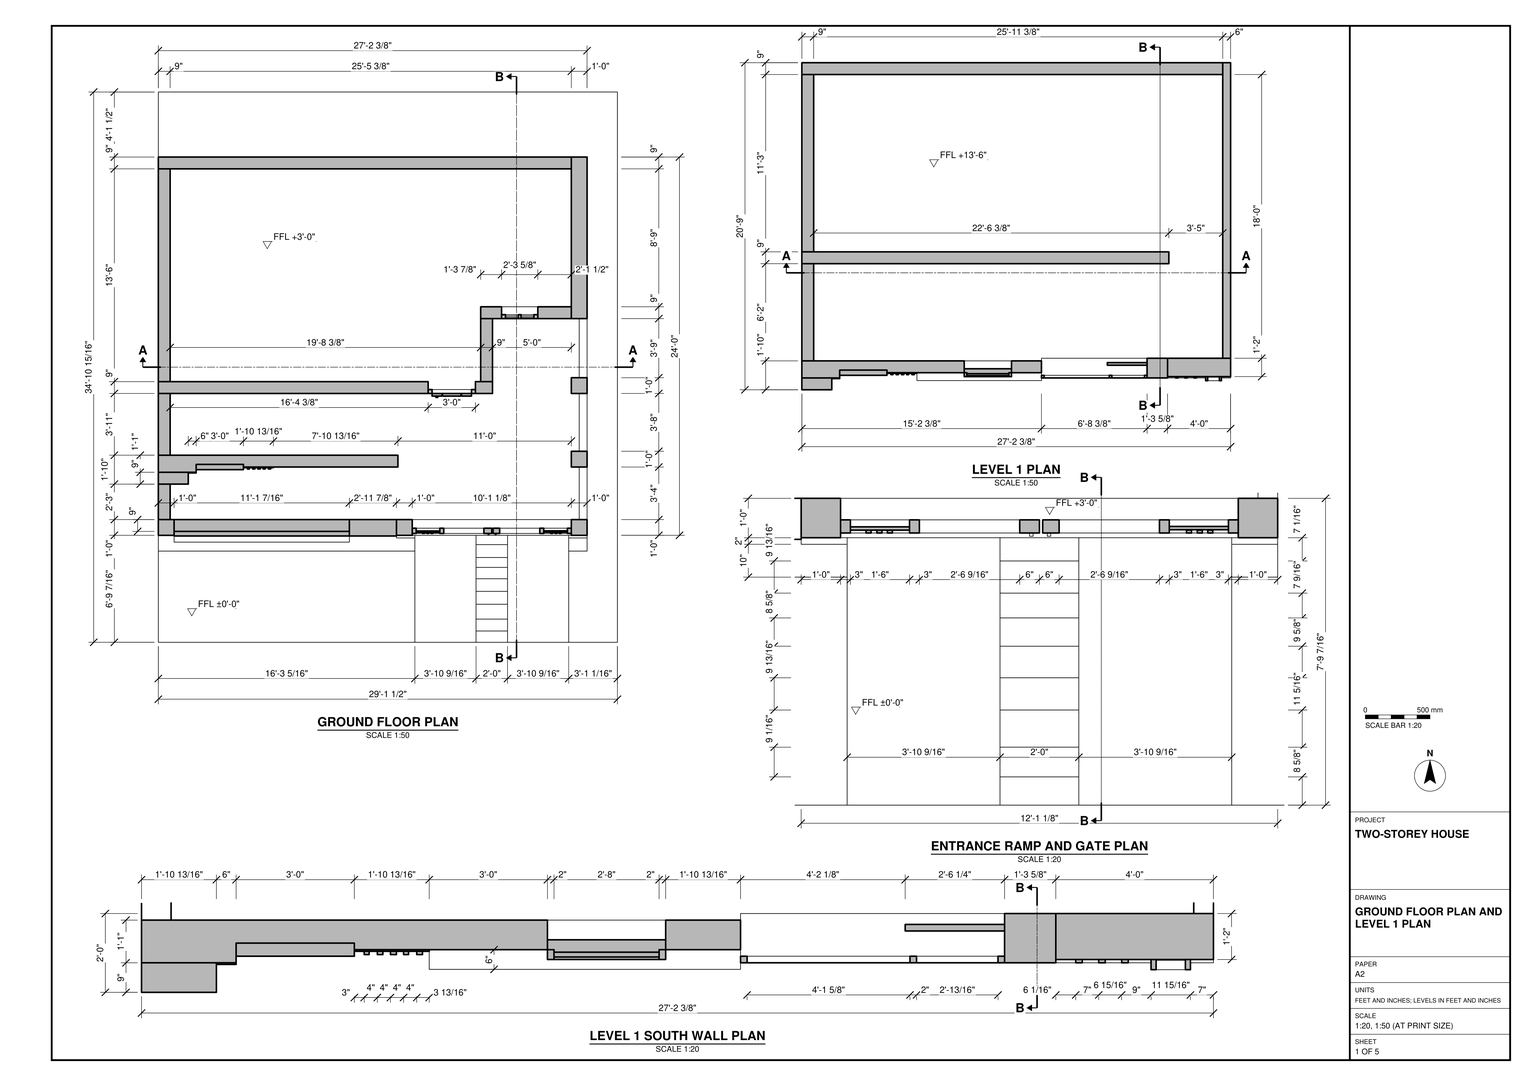
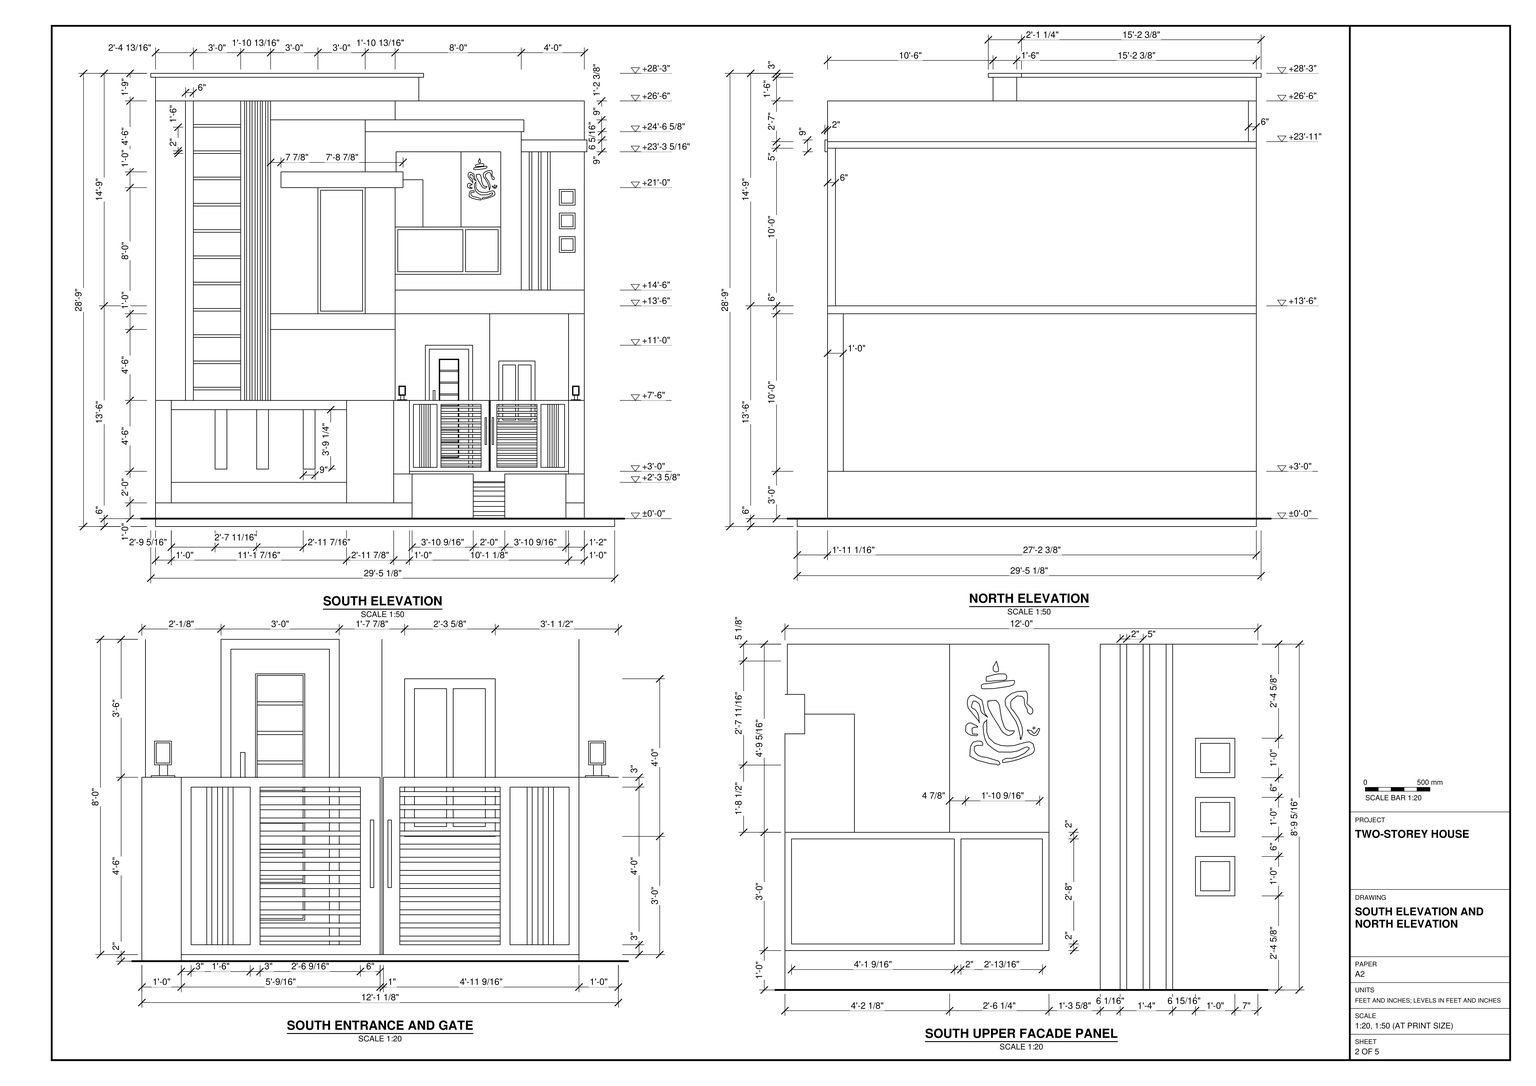
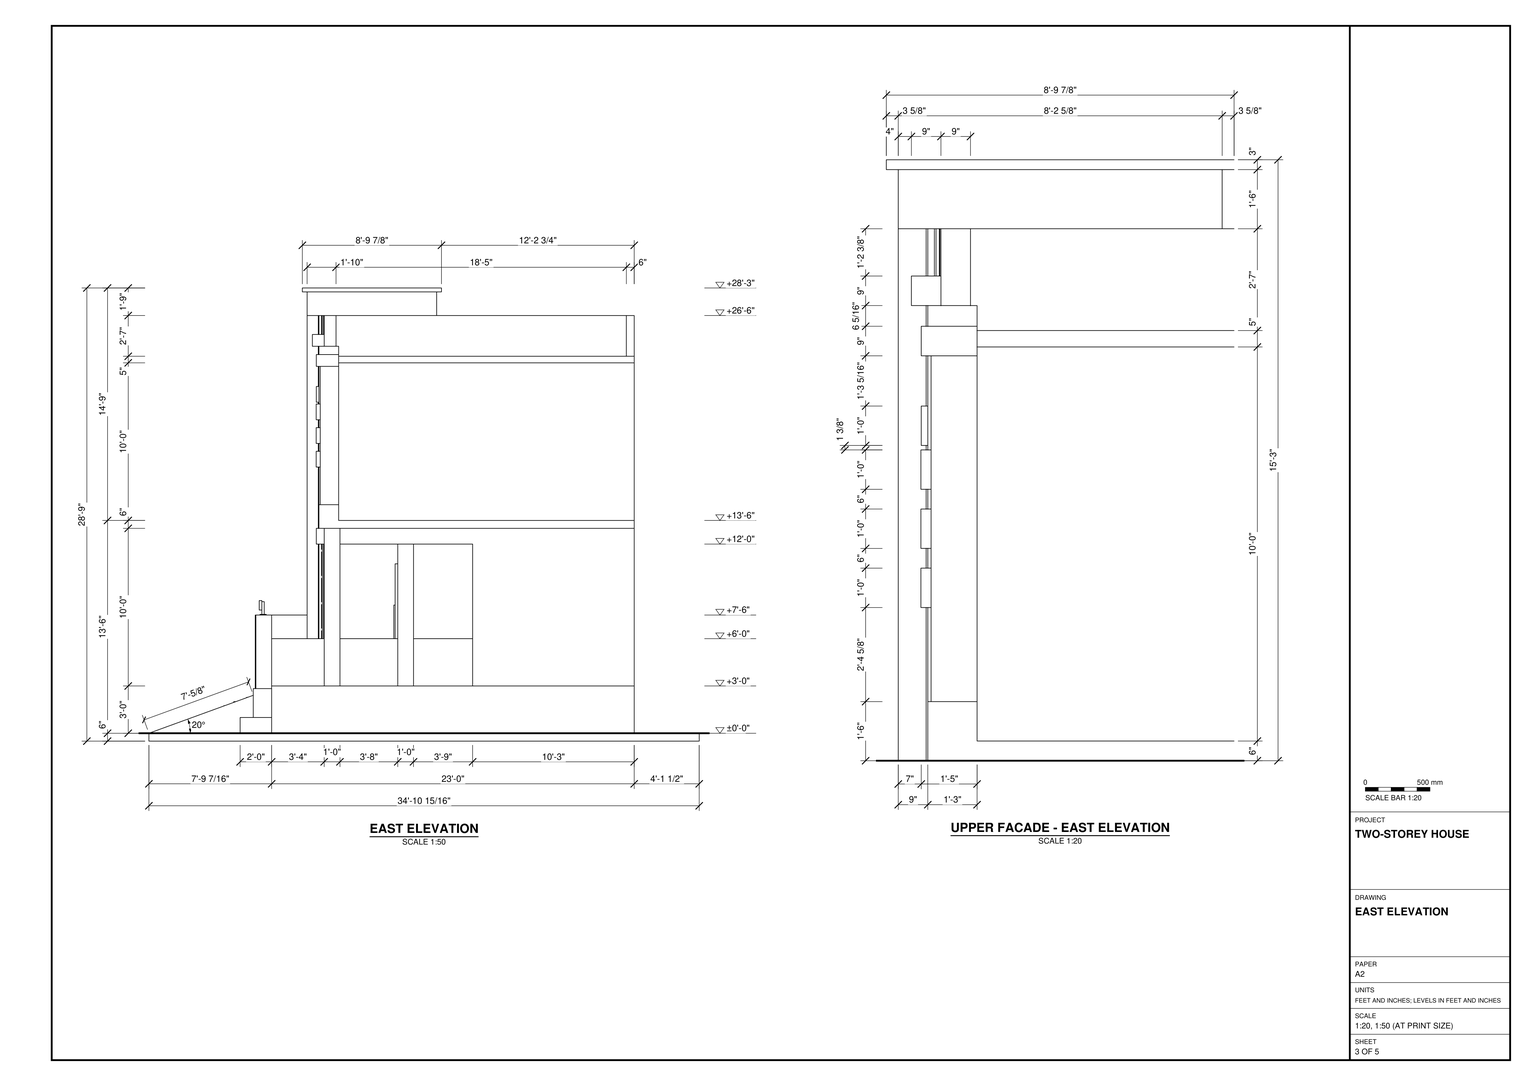
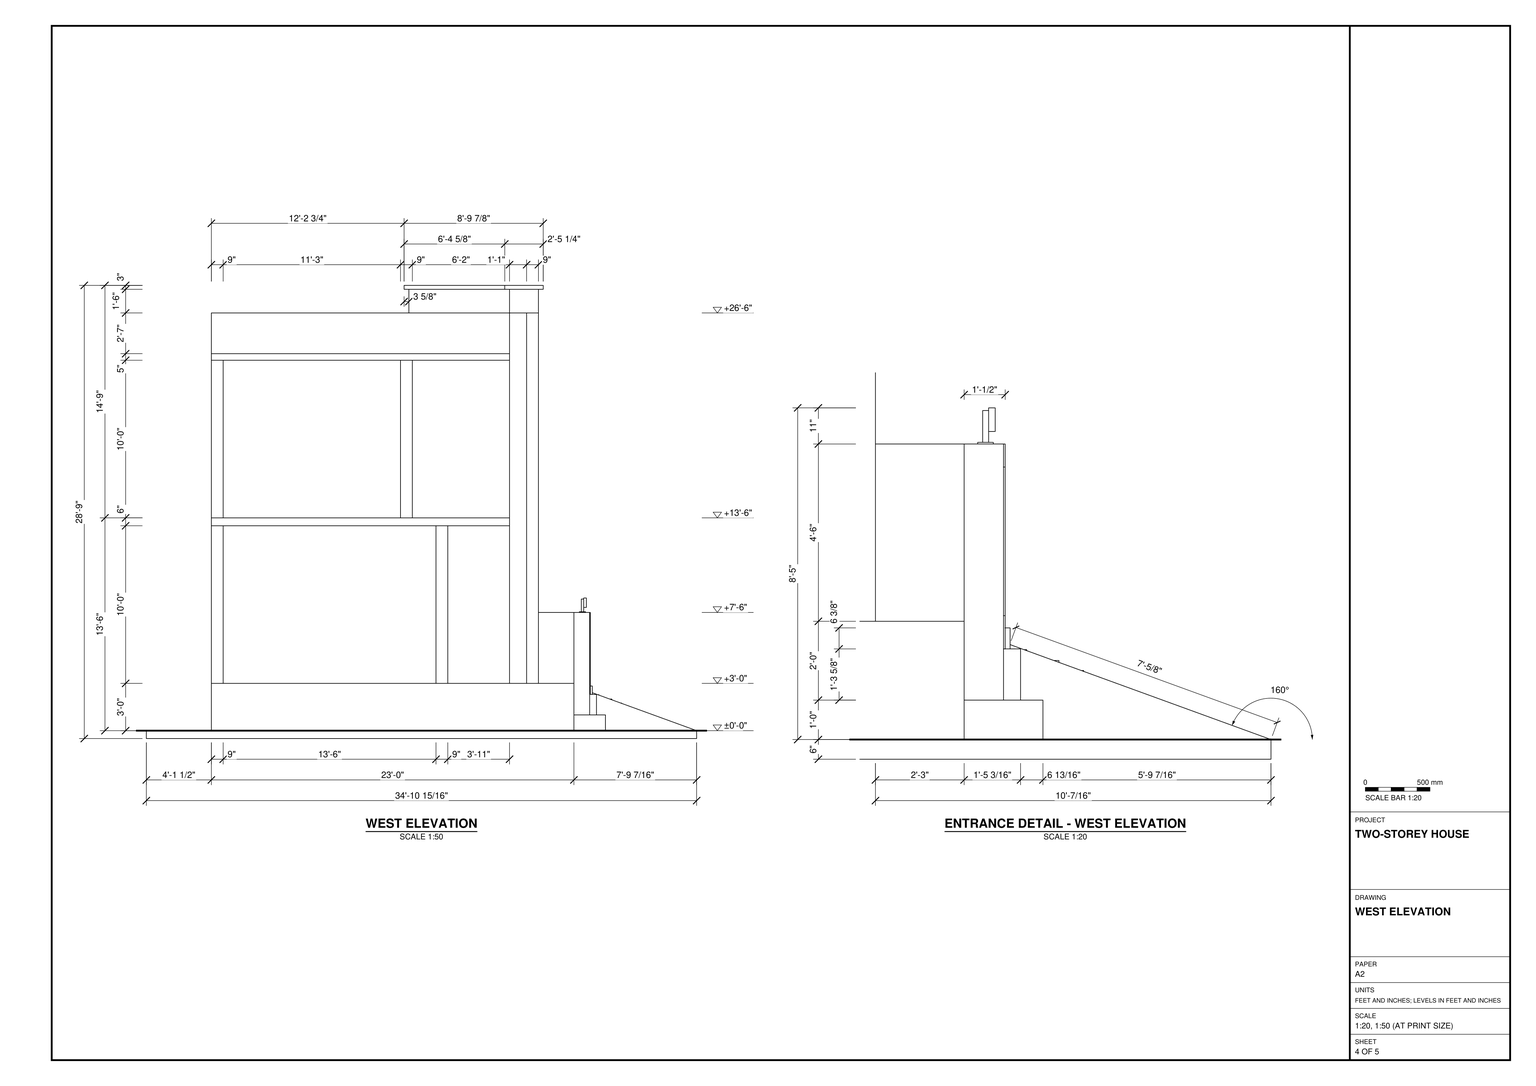
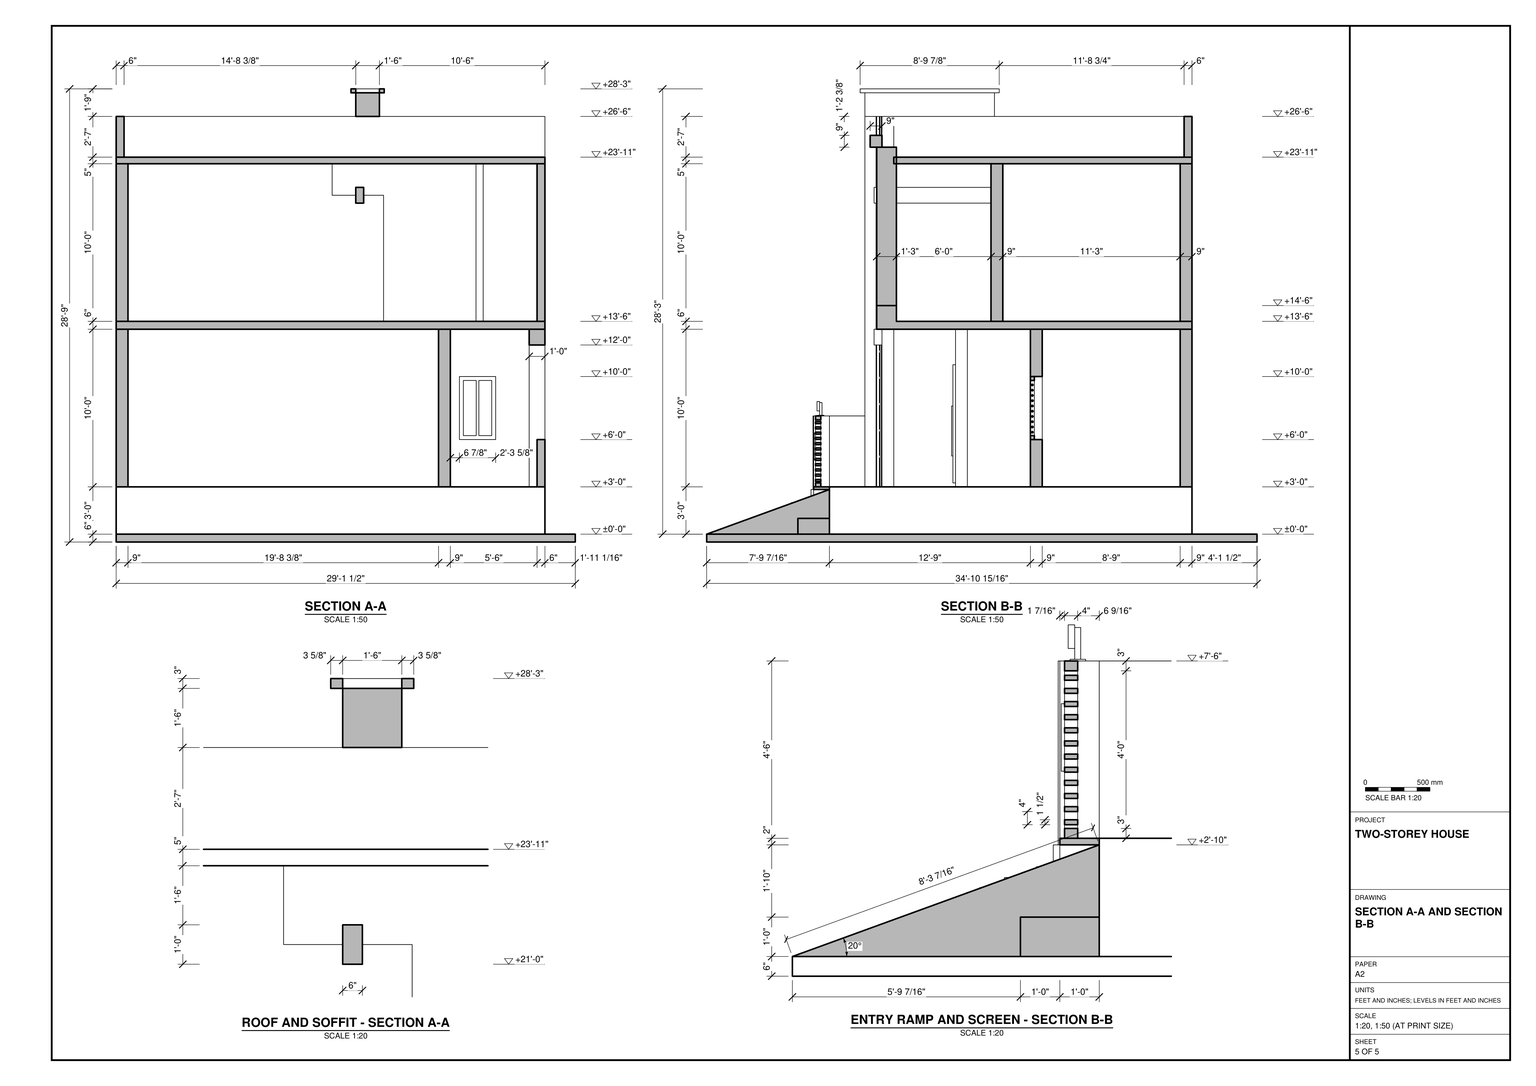
Build the house shown in task_files/diagram_01.pdf in SketchUp. Work in feet and inches, with the south entrance facing the front of the site. Including the base and projecting elements, the overall model must be 29'-5 1/8" wide, 34'-10 15/16" deep and 28'-9" high. Use ±0'-0" as the ground datum and +13'-6" as the upper floor level. The raised lower floor and entrance landing are at +3'-0".

Follow the plans for wall thicknesses, returns, partitions and openings. Model the broad rear room, the recessed entrance area with its posts, and the upper floor with its cross-wall stopping short of the east wall. Include the base, floor slabs, flat roof, parapets and projecting caps. At the south entrance, run the central steps and flanking ramps up to the slatted gate. Set the entrance door and adjacent window back from the gate as drawn.

Use the south elevation for the arrangement of openings, fins and framed panels, and the east elevation for the depths of the projecting bands and hoods. Decor and loose items shown may be represented by any suitable library components. Keep walls, slabs, roof and each furniture or joinery piece shown as separate groups or components, and use components for repeated parts. Save one SketchUp model as output_files/two_storey_house_with_a_gated_entrance.skp.

# SketchUp Ruby script. Lengths in inches.
U = 1.inch
M = Sketchup.active_model
def pt(a) = Geom::Point3d.new(a.map { |v| v * U })
def face(e, loops, mat)
  f = e.add_face(loops[0].map { |a| pt(a) })
  loops[1..].each { |l| e.add_face(l.map { |a| pt(a) }).erase! }
  f.material = f.back_material = mat if mat
  f
end
# faces: each face lists its corners as indices into pts; further lists are holes
def faces(e, pts, list, mat = nil) = list.each { |f| face(e, (f[0].is_a?(Array) ? f : [f]).map { |l| l.map { |i| pts[i] } }, mat) }
# xy, xz, yz: faces in a plane at the given z, y or x. An outline is a flat list of corners, or four numbers for a rectangle; further outlines are holes
def ring(l) = l.size == 4 ? [[l[0], l[1]], [l[2], l[1]], [l[2], l[3]], [l[0], l[3]]] : l.each_slice(2).to_a
def flat(e, list, mat, &to3) = list.each { |f| face(e, (f[0].is_a?(Array) ? f : [f]).map { |l| ring(l).map { |u, v| to3.(u, v) } }, mat) }
def xy(e, z, list, mat = nil) = flat(e, list, mat) { |x, y| [x, y, z] }
def xz(e, y, list, mat = nil) = flat(e, list, mat) { |x, z| [x, y, z] }
def yz(e, x, list, mat = nil) = flat(e, list, mat) { |y, z| [x, y, z] }
def lines(e, pts, list) = list.each { |a, b| e.add_line(pt(pts[a]), pt(pts[b])) }
# prism: a flat outline (further loops are holes) pulled along v
def prism(e, loops, v, mat = nil)
  f = face(e, loops, mat); d = Geom::Vector3d.new(v.map { |x| x * U })
  f.pushpull(f.normal.samedirection?(d) ? d.length : -d.length)
end
def box(e, o, s, mat = nil) = prism(e, [[o, [o[0] + s[0], o[1], o[2]], [o[0] + s[0], o[1] + s[1], o[2]], [o[0], o[1] + s[1], o[2]]]], [0, 0, s[2]], mat)
def at(x, y, z, deg = 0) = Geom::Transformation.translation(pt([x, y, z])) * Geom::Transformation.rotation(ORIGIN, Z_AXIS, deg.degrees)
def axes(o, x, y, z) = Geom::Transformation.new([*x, 0, *y, 0, *z, 0, *pt(o).to_a, 1])
def part(name) = M.definitions.add(name)
# library, detail: a bought-in or finely detailed component or shape, given as its bounding box
def library(name, o, s) = part(name).tap { |d| box(d.entities, o, s) }
def detail(e, o, s) = box(e.add_group.entities, o, s)
def put(e, d, t, mat = nil) = e.add_instance(d, t).tap { |i| i.material = mat if mat }
def group(e, t, mat = nil) = e.add_group.tap { |g| g.transformation = t; g.material = mat if mat }.entities
root = M.entities
M.materials.add("[Blacktop New]").color = [30, 30, 30]
M.materials.add("[Brick Antique 01]2").color = [147, 30, 30]
M.materials.add("[Color A07]").color = [109, 0, 0]
M.materials.add("[Color A07]1").color = [153, 0, 0]
M.materials.add("[Color A08]").color = [102, 0, 0]
M.materials.add("[Color D03]").color = [255, 216, 101]
M.materials.add("[Color E03]").color = [255, 255, 101]
M.materials.add("[Color M00]").color = [255, 255, 255]
M.materials.add("[Color M09]").color = [0, 0, 0]
M.materials.add("[Metal Aluminum Anodized]").color = [202, 209, 219]
M.materials.add("[Polished Concrete New]").color = [200, 200, 203]
M.materials.add("[Translucent Glass Gray]").color = [0, 0, 0]
M.materials["[Translucent Glass Gray]"].alpha = 0.5
c1 = part("Group\#8")
prism(c1.entities,[[[21.6,0.07,0.75],[21.6,0.02,0.63],[21.6,0,0.5],[21.6,0.02,0.37],[21.6,0.07,0.25],[21.6,0.15,0.15],[21.6,0.25,0.07],[21.6,0.37,0.02],[21.6,0.5,0],[21.6,0.63,0.02],[21.6,0.75,0.07],[21.6,0.85,0.15],[21.6,0.93,0.25],[21.6,0.98,0.37],[21.6,1,0.5],[21.6,0.98,0.63],[21.6,0.93,0.75],[21.6,0.85,0.85],[21.6,0.75,0.93],[21.6,0.63,0.98],[21.6,0.5,1],[21.6,0.37,0.98],[21.6,0.25,0.93],[21.6,0.15,0.85]]],[-21.6,0,0])
c2 = part("Group\#17")
prism(c2.entities,[[[32,1.5,0.75],[32,1.47,0.94],[32,1.4,1.125],[32,1.28,1.28],[32,1.125,1.4],[32,0.94,1.47],[32,0.75,1.5],[32,0.56,1.47],[32,0.375,1.4],[32,0.22,1.28],[32,0.1,1.125],[32,0.03,0.94],[32,0,0.75],[32,0.03,0.56],[32,0.1,0.375],[32,0.22,0.22],[32,0.375,0.1],[32,0.56,0.03],[32,0.75,0],[32,0.94,0.03],[32,1.125,0.1],[32,1.28,0.22],[32,1.4,0.375],[32,1.47,0.56]]],[-32,0,0])
c3 = part("Group\#31")
box(c3.entities,[0,0,0],[2,1,105.3])
c4 = part("Group\#67")
box(c4.entities,[0,0,0],[30.55,4,1.5])
c5 = part("Group\#68")
put(c5.entities,c4,at(0,0,44))
put(c5.entities,c4,at(0,0,32))
put(c5.entities,c4,at(0,0,24))
put(c5.entities,c4,at(0,0,12))
put(c5.entities,c4,at(0,0,28))
put(c5.entities,c4,at(0,0,36))
put(c5.entities,c4,at(0,0,16))
put(c5.entities,c4,at(0,0,40))
put(c5.entities,c4,at(0,0,8))
put(c5.entities,c4,at(0,0,20))
put(c5.entities,c4,at(0,0,4))
put(c5.entities,c4,at(0,0,0))
c6 = part("Group\#71")
box(c6.entities,[0,0,0],[1.54,0.875,48])
c7 = part("Group\#72")
put(c7.entities,c6,at(6.49,0,0))
put(c7.entities,c6,at(0,0,0))
put(c7.entities,c6,at(3.3,0,0))
c8 = part("Group\#74")
prism(c8.entities,[[[46.55,93.4375,0],[46.55,93.4375,34],[46.55,0,0],[46.55,69.4375,0]]],[-46.55,0,0])
c9 = part("Group\#84")
box(c9.entities,[0,0,0],[1.0625,1,20.5625])
c10 = library("Group\#47",[0,0,0],[22.59,2.125,31.69])
c11 = part("Group\#91")
xy(c11.entities,0,[[0,0,7.1875,4.75]])
xy(c11.entities,0.5,[[[0,0,7.1875,4.75],[2.48,1.42,4.98,3.23]]])
xy(c11.entities,10.1875,[[2.48,1.42,4.98,3.23]])
xz(c11.entities,0,[[0,0,7.1875,0.5]])
xz(c11.entities,1.42,[[2.48,0.5,4.98,3.8],[2.48,3.8,4.98,10.1875]])
xz(c11.entities,3.23,[[2.48,0.5,4.98,10.1875]])
xz(c11.entities,4.75,[[0,0,7.1875,0.5]])
yz(c11.entities,0,[[0,0,4.75,0.5]])
yz(c11.entities,2.48,[[1.42,0.5,3.23,10.1875]])
yz(c11.entities,4.98,[[1.42,0.5,3.23,10.1875]])
yz(c11.entities,7.1875,[[0,0,4.75,0.5]])
prism(root,[[[99.13,133.4375,258],[186.04,133.4375,258],[186.04,216.4375,258],[192.04,216.4375,258],[192.04,127.4375,258],[99.13,127.4375,258]]],[0,0,12])
xy(root,42,[[3.64,142.4375,12.64,189.4375]])
xy(root,162,[[3.64,142.4375,12.64,189.4375]])
xz(root,142.4375,[[3.64,42,12.64,162]])
xz(root,189.4375,[[3.64,42,12.64,162]])
yz(root,12.64,[[142.4375,42,189.4375,162]])
p = [[186.04,133.4375,258],[186.04,133.4375,257.875],[198.93,69.4375,6],[198.93,69.4375,18],[198.93,79.4375,18],[316.04,69.4375,6],
  [316.04,69.4375,18],[316.04,79.4375,18]]
lines(root,p,[[0,1],[2,3],[3,4],[5,6],[6,7]])
g1 = group(root,at(-29.96,189.4375,42))
prism(g1,[[[288,9,0],[275,9,0],[275,9,96],[239,9,96],[239,9,0],[33.6,9,0],[33.6,9,120],[288,9,120]]],[0,-9,0])
g2 = group(root,at(249.04,198.4375,42))
box(g2,[0,0,0],[9,48,120])
g3 = group(root,at(249.04,246.4375,42))
prism(g3,[[[69,9,0],[0,9,0],[0,9,120],[69,9,120]],[[15.9,9,36],[43.5,9,36],[43.5,9,84],[15.9,9,84]]],[0,-9,0])
g4 = group(root,at(318.04,246.4375,42))
prism(g4,[[[12,0,0],[12,123,0],[12,123,120],[12,-101,120],[12,-101,108],[12,0,108]]],[-12,0,0])
g5 = group(root,at(-29.96,360.4375,42))
box(g5,[33.6,0,0],[314.4,9,120])
g6 = group(root,at(264.9375,246.4375,78),"[Color M09]")
prism(g6,[[[27.6,3,0],[0,3,0],[0,3,48],[27.6,3,48]],[[12.8,3,3],[12.8,3,45],[3,3,45],[3,3,3]],[[24.6,3,45],[14.8,3,45],[14.8,3,3],[24.6,3,3]]],[0,-3,0])
g7 = group(root,at(267.9375,247.4375,83.1))
put(g7,c1,at(0,0,28))
put(g7,c1,at(0,0,36))
put(g7,c1,at(0,0,24))
put(g7,c1,at(0,0,16))
put(g7,c1,at(0,0,12))
put(g7,c1,at(0,0,20))
put(g7,c1,at(0,0,32))
put(g7,c1,at(0,0,0))
put(g7,c1,at(0,0,8))
put(g7,c1,at(0,0,4))
g8 = group(root,at(279.74,246.4375,81),"[Translucent Glass Gray]")
xz(g8,0,[[0,0,9.8,42]])
g9 = group(root,at(267.9375,246.4375,81),"[Translucent Glass Gray]")
xz(g9,0,[[0,0,9.8,42]])
g10 = group(root,at(209.04,189.4375,42),"[Color A07]")
prism(g10,[[[0,0,96],[0,0,0],[36,0,0],[36,0,96]],[[33,0,93],[33,0,3],[3,0,3],[3,0,93]]],[0,3,0])
g11 = group(root,at(212.04,187.4375,45),"[Color A07]")
xy(g11,0,[[0,0,30,2]])
xy(g11,7.5,[[7.5,0,22.5,1]])
xy(g11,8,[[8,0,22,1]])
xy(g11,19,[[8,0,22,0.5]])
xy(g11,20,[[8,0,22,0.5]])
xy(g11,28,[[8,0,22,0.5]])
xy(g11,29,[[8,0,22,0.5]])
xy(g11,37,[[8,0,22,0.5]])
xy(g11,38,[[8,0,22,0.5]])
xy(g11,46,[[8,0,22,0.5]])
xy(g11,47,[[8,0,22,0.5]])
xy(g11,55,[[8,0,22,0.5]])
xy(g11,56,[[8,0,22,0.5]])
xy(g11,64,[[8,0,22,0.5]])
xy(g11,65,[[8,0,22,0.5]])
xy(g11,73,[[8,0,22,0.5]])
xy(g11,74,[[8,0,22,0.5]])
xy(g11,82,[[8,0,22,1]])
xy(g11,82.5,[[7.5,0,22.5,1]])
xy(g11,90,[[0,0,30,2]])
xz(g11,0,[[[0,0,30,90],[7.5,7.5,22.5,82.5]],[8,8,22,19],[8,20,22,28],[8,29,22,37],[8,38,22,46],
  [8,47,22,55],[8,56,22,64],[8,65,22,73],[8,74,22,82]])
xz(g11,0.5,[[8,19,22,20],[8,28,22,29],[8,37,22,38],[8,46,22,47],[8,55,22,56],
  [8,64,22,65],[8,73,22,74]])
xz(g11,1,[[[7.5,7.5,22.5,82.5],[8,8,22,82]]])
xz(g11,2,[[0,0,30,90]])
yz(g11,0,[[0,0,2,90]])
yz(g11,7.5,[[0,7.5,1,82.5]])
yz(g11,8,[[0,8,0,19,0.5,19,0.5,20,0,20,0,28,0.5,28,0.5,29,0,29,0,37,0.5,37,0.5,38,0,38,0,46,0.5,46,0.5,47,0,47,0,55,0.5,55,0.5,56,0,56,0,64,0.5,64,0.5,65,0,65,0,73,0.5,73,0.5,74,0,74,0,82,1,82,1,8]])
yz(g11,22,[[0,8,1,8,1,82,0,82,0,74,0.5,74,0.5,73,0,73,0,65,0.5,65,0.5,64,0,64,0,56,0.5,56,0.5,55,0,55,0,47,0.5,47,0.5,46,0,46,0,38,0.5,38,0.5,37,0,37,0,29,0.5,29,0.5,28,0,28,0,20,0.5,20,0.5,19,0,19]])
yz(g11,22.5,[[0,7.5,1,82.5]])
yz(g11,30,[[0,0,2,90]])
g12 = group(root,at(-29.96,189.4375,162))
xy(g12,0,[[216,-60,216,-47,33.6,-47,33.6,180,360,180,360,-60]])
xy(g12,6,[[33.6,-47,216,-47,216,-45,360,-45,360,180,33.6,180]])
xy(g12,18,[[216,-60,360,-45]])
xz(g12,-60,[[216,0,360,18]])
xz(g12,-47,[[33.6,0,216,6]])
xz(g12,-45,[[216,6,360,18]])
xz(g12,180,[[33.6,0,360,6]])
yz(g12,33.6,[[-47,0,180,6]])
yz(g12,216,[[-60,0,-60,18,-51,18,-51,6,-47,6,-47,0],[-51,6,-45,18]])
yz(g12,360,[[-60,0,180,0,180,6,-45,6,-45,18,-60,18]])
g13 = group(root,at(-29.96,129.4375,42))
xy(g13,0,[[33.6,0,33.6,13,216,13,216,4,98.4,4,98.4,6,62.4,6,62.4,0]])
xy(g13,120,[[157.2,4,193.2,7],[157.2,7,193.2,13]])
xy(g13,216,[[157.2,4,193.2,7],[157.2,7,193.2,13]])
xy(g13,282,[[33.6,0,62.4,0,62.4,6,98.4,6,98.4,4,216,4,216,13,33.6,13]])
xz(g13,0,[[33.6,0,62.4,282]])
xz(g13,4,[[[98.4,0,216,282],[157.2,120,193.2,216]]])
xz(g13,6,[[62.4,0,98.4,282]])
xz(g13,7,[[157.2,120,193.2,216]],"[Color M00]")
xz(g13,13,[[[33.6,0,216,282],[157.2,120,193.2,216]]])
yz(g13,33.6,[[0,0,13,282]])
yz(g13,62.4,[[0,0,6,282]])
yz(g13,98.4,[[4,0,6,282]])
yz(g13,157.2,[[4,120,7,216],[7,120,13,216]])
yz(g13,193.2,[[4,120,7,216],[7,120,13,216]])
yz(g13,216,[[4,0,13,282]])
g14 = group(root,at(127.24,130.4375,162),"[Color M09]")
g15 = group(g14,at(2,0.75,4.64),"[Metal Aluminum Anodized]")
put(g15,c2,at(0,0,54))
put(g15,c2,at(0,0,12))
put(g15,c2,at(0,0,0))
put(g15,c2,at(0,0,42))
put(g15,c2,at(0,0,48))
put(g15,c2,at(0,0,6))
put(g15,c2,at(0,0,30))
put(g15,c2,at(0,0,18))
put(g15,c2,at(0,0,24))
put(g15,c2,at(0,0,36))
put(g15,c2,at(0,0,84))
put(g15,c2,at(0,0,60))
put(g15,c2,at(0,0,78))
put(g15,c2,at(0,0,72))
put(g15,c2,at(0,0,66))
g16 = group(g14,at(0,0,0))
prism(g16,[[[36,0,0],[36,0,96],[0,0,96],[0,0,0]],[[2,0,94],[34,0,94],[34,0,2],[2,0,2]]],[0,3,0])
g17 = group(root,at(129.24,130.4375,164),"[Translucent Glass Gray]")
xz(g17,0,[[0,0,32,92]],"[Translucent Glass Gray]")
g18 = group(root,at(32.4375,132.4375,42),"[Polished Concrete New]")
prism(g18,[[[36,3,0],[36,3,282],[36,-1,282],[36,-1,264],[36,-0.5,264],[36,-0.5,262],[36,-1,262],[36,-1,244],[36,-0.5,244],[36,-0.5,242],[36,-1,242],[36,-1,224],[36,-0.5,224],[36,-0.5,222],[36,-1,222],[36,-1,204],[36,-0.5,204],[36,-0.5,202],[36,-1,202],[36,-1,184],[36,-0.5,184],[36,-0.5,182],[36,-1,182],[36,-1,164],[36,-0.5,164],[36,-0.5,162],[36,-1,162],[36,-1,144],[36,-0.5,144],[36,-0.5,142],[36,-1,142],[36,-1,124],[36,-0.5,124],[36,-0.5,122],[36,-1,122],[36,-1,104],[36,-0.5,104],[36,-0.5,102],[36,-1,102],[36,-1,84],[36,-0.5,84],[36,-0.5,82],[36,-1,82],[36,-1,64],[36,-0.5,64],[36,-0.5,62],[36,-1,62],[36,-1,44],[36,-0.5,44],[36,-0.5,42],[36,-1,42],[36,-1,24],[36,-0.5,24],[36,-0.5,22],[36,-1,22],[36,-1,0]]],[-36,0,0])
g19 = group(root,at(-29.96,129.4375,30))
box(g19,[33.6,-36,-24],[326.4,276,36])
g20 = group(root,at(26.4375,128.9375,42),"[Color A07]")
box(g20,[0,0,0],[6,0.5,282])
g21 = group(root,at(68.4375,132.9375,42))
box(g21,[0,0,0],[22.8,0.5,282],"[Color A07]")
g22 = group(root,at(71.4375,131.9375,42))
box(g22,[0,0,0],[1.5,1,282])
g23 = group(root,at(75.4375,131.9375,42))
box(g23,[0,0,0],[1.6875,1,282])
g24 = group(root,at(79.4375,131.9375,42))
box(g24,[0,0,0],[1.8125,1,282])
g25 = group(root,at(83.4375,131.9375,42))
box(g25,[0,0,0],[1.5,1,282])
g26 = group(root,at(87.4375,131.9375,42))
box(g26,[0,0,0],[1.75,1,282])
g27 = group(root,at(91.24,127.4375,150))
box(g27,[0,0,0],[94.8,6,12])
g28 = group(root,at(163.24,128.4375,270),"[Color A07]")
prism(g28,[[[0,16,30.6],[118.8,16,30.6],[118.8,16,-90],[22.8,16,-90],[22.8,16,-78],[103.2,16,-78],[103.2,16,15.3],[23.53,16,15.3],[23.53,16,0],[0,16,0]]],[0,-15,0])
g29 = group(root,at(282.04,130.4375,180))
box(g29,[0,0,0],[48,14,105.3],"[Color A07]")
g30 = group(root,at(163.24,124.4375,300.6))
box(g30,[0,0,0],[120.8,9,9])
g31 = group(root,at(282.04,127.4375,285.3))
box(g31,[0,0,0],[50,17,9])
put(root,c3,at(288.1,129.4375,180))
put(root,c3,at(295.1,129.4375,180))
put(root,c3,at(302.1,129.4375,180))
g32 = group(root,at(311.04,127.34,226.65))
xy(g32,0,[[0,0,12,3.1]])
xy(g32,1.55,[[1.55,0,10.45,3]])
xy(g32,10.45,[[1.55,0,10.45,3]])
xy(g32,12,[[0,0,12,3.1]])
xz(g32,0,[[[0,0,12,12],[1.55,1.55,10.45,10.45]]])
xz(g32,3,[[1.55,1.55,10.45,10.45]],"[Color D03]")
xz(g32,3.1,[[[0,0,12,12],[1.55,1.55,10.45,10.45]]])
yz(g32,0,[[0,0,3.1,12]])
yz(g32,1.55,[[0,1.55,3,10.45]])
yz(g32,10.45,[[0,1.55,3,10.45]])
yz(g32,12,[[0,0,3.1,12]])
p = [[10.45,3.1,10.45],[10.45,3,10.45],[1.55,3.1,1.55],[1.55,3,1.55],[1.55,3.1,10.45],[1.55,3,10.45],
  [10.45,3.1,1.55],[10.45,3,1.55]]
lines(g32,p,[[0,1],[2,3],[4,5],[6,7]])
g33 = group(root,at(311.04,127.34,208.65))
xy(g33,0,[[0,0,12,3.1]],"[Color D03]")
xy(g33,1.55,[[1.55,0,10.45,3]],"[Color D03]")
xy(g33,10.45,[[1.55,0,10.45,3]],"[Color D03]")
xy(g33,12,[[0,0,12,3.1]],"[Color D03]")
xz(g33,0,[[[0,0,12,12],[1.55,1.55,10.45,10.45]]],"[Color D03]")
xz(g33,3,[[1.55,1.55,10.45,10.45]],"[Color D03]")
xz(g33,3.1,[[[0,0,12,12],[1.55,1.55,10.45,10.45]]],"[Color D03]")
yz(g33,0,[[0,0,3.1,12]],"[Color D03]")
yz(g33,1.55,[[0,1.55,3,10.45]],"[Color D03]")
yz(g33,10.45,[[0,1.55,3,10.45]],"[Color D03]")
yz(g33,12,[[0,0,3.1,12]],"[Color D03]")
p = [[10.45,3.1,10.45],[10.45,3,10.45],[1.55,3.1,1.55],[1.55,3,1.55],[1.55,3.1,10.45],[1.55,3,10.45],
  [10.45,3.1,1.55],[10.45,3,1.55]]
lines(g33,p,[[0,1],[2,3],[4,5],[6,7]])
g34 = group(root,at(311.04,127.34,244.65))
xy(g34,0,[[0,0,12,3.1]])
xy(g34,1.55,[[1.55,0,10.45,3]])
xy(g34,10.45,[[1.55,0,10.45,3]])
xy(g34,12,[[0,0,12,3.1]])
xz(g34,0,[[[0,0,12,12],[1.55,1.55,10.45,10.45]]])
xz(g34,3,[[1.55,1.55,10.45,10.45]],"[Color D03]")
xz(g34,3.1,[[[0,0,12,12],[1.55,1.55,10.45,10.45]]])
yz(g34,0,[[0,0,3.1,12]])
yz(g34,1.55,[[0,1.55,3,10.45]])
yz(g34,10.45,[[0,1.55,3,10.45]])
yz(g34,12,[[0,0,3.1,12]])
p = [[10.45,3.1,10.45],[10.45,3,10.45],[1.55,3.1,1.55],[1.55,3,1.55],[1.55,3.1,10.45],[1.55,3,10.45],
  [10.45,3.1,1.55],[10.45,3,1.55]]
lines(g34,p,[[0,1],[2,3],[4,5],[6,7]])
g35 = group(root,at(91.24,133.14,309.6),"[Color A07]")
box(g35,[0,0,0],[94.8,0.3,14.4])
g36 = group(root,at(3.64,120.4375,42))
box(g36,[0,0,0],[22.8,9,282])
g37 = group(root,at(0,116.8,324))
xy(g37,0,[[3.64,3.64,3.64,25.64,186.04,25.64,186.04,102.26,204.04,102.26,204.04,3.64]])
xy(g37,18,[[[0,0,0,29.27,182.4,29.27,182.4,105.9,207.67,105.9,207.67,0],[3.64,3.64,204.04,3.64,204.04,102.26,186.04,102.26,186.04,25.64,3.64,25.64]],[3.64,3.64,204.04,3.64,204.04,102.26,186.04,102.26,186.04,25.64,3.64,25.64]])
xy(g37,21,[[[0,0,207.67,0,207.67,105.9,182.4,105.9,182.4,29.27,0,29.27],[3.64,3.64,3.64,25.64,186.04,25.64,186.04,102.26,204.04,102.26,204.04,3.64]]],"[Color A08]")
xz(g37,0,[[0,18,207.67,21]],"[Color A08]")
xz(g37,3.64,[[3.64,0,204.04,18]])
xz(g37,3.64,[[3.64,18,204.04,21]],"[Color A08]")
xz(g37,25.64,[[3.64,0,186.04,18]])
xz(g37,25.64,[[3.64,18,186.04,21]],"[Color A08]")
xz(g37,29.27,[[0,18,182.4,21]],"[Color A08]")
xz(g37,102.26,[[186.04,0,204.04,18]])
xz(g37,102.26,[[186.04,18,204.04,21]],"[Color A08]")
xz(g37,105.9,[[182.4,18,207.67,21]])
yz(g37,0,[[0,18,29.27,21]],"[Color A08]")
yz(g37,3.64,[[3.64,0,25.64,18],[3.64,18,25.64,21]])
yz(g37,182.4,[[29.27,18,105.9,21]],"[Color A08]")
yz(g37,186.04,[[25.64,0,102.26,18]])
yz(g37,186.04,[[25.64,18,102.26,21]],"[Color A08]")
yz(g37,204.04,[[3.64,0,102.26,18]])
yz(g37,204.04,[[3.64,18,102.26,21]],"[Color A08]")
yz(g37,207.67,[[0,18,105.9,21]],"[Color A08]")
g38 = group(root,at(3.64,216.4375,168))
xy(g38,0,[[0,0,279.39,9]])
xy(g38,120,[[0,0,279.39,9]])
xz(g38,0,[[0,0,203.55,0,203.55,96,164.4,96,164.4,120,0,120],[273.93,0,279.39,120]])
xz(g38,0,[[203.55,0,273.93,0,273.93,120,164.4,120,164.4,96,203.55,96]],"[Brick Antique 01]2")
xz(g38,9,[[0,0,279.39,120]])
yz(g38,0,[[0,0,9,120]])
yz(g38,279.39,[[0,0,9,120]])
g39 = group(root,at(3.64,144.4375,168))
xy(g39,0,[[320.4,0,326.4,225],[0,216,320.4,225]])
xy(g39,120,[[320.4,0,326.4,225],[0,216,320.4,225]])
xz(g39,0,[[320.4,0,326.4,120]])
xz(g39,216,[[0,0,320.4,120]])
xz(g39,225,[[0,0,320.4,120],[320.4,0,326.4,120]])
yz(g39,0,[[216,0,225,120]])
yz(g39,320.4,[[0,0,216,120],[216,0,225,120]])
yz(g39,326.4,[[0,0,225,120]])
g40 = group(root,at(3.64,225.4375,168))
box(g40,[0,0,0],[9,135,120])
g41 = group(root,at(3.64,198.4375,42))
box(g41,[0,0,0],[9,162,120])
g42 = group(root,at(3.64,142.4375,42))
yz(g42,0,[[0,0,47,120]])
g43 = group(root,at(3.64,142.4375,168))
box(g43,[0,0,0],[9,74,120])
g44 = group(root,at(3.64,142.4375,288))
xy(g44,0,[[0,0,326.4,227]],"[Color E03]")
xy(g44,5,[[0,0,326.4,227]])
xz(g44,0,[[0,0,326.4,5]])
xz(g44,227,[[0,0,326.4,5]])
yz(g44,0,[[0,0,227,5]])
yz(g44,326.4,[[0,0,227,5]])
g45 = group(root,at(186.04,129.4375,192),"[Color M09]")
prism(g45,[[[0,2,0],[0,2,36],[80.4,2,36],[80.4,2,0]],[[51.59,2,34],[2,2,34],[2,2,2],[51.59,2,2]],[[53.59,2,34],[53.59,2,2],[78.4,2,2],[78.4,2,34]]],[0,-2,0])
g46 = group(root,at(239.625,129.4375,194),"[Translucent Glass Gray]")
xz(g46,0,[[0,0,24.81,32]])
g47 = group(root,at(188.04,129.4375,194),"[Translucent Glass Gray]")
xz(g47,0,[[0,0,49.59,32]])
g48 = group(root,at(318.04,133.4375,42))
box(g48,[0,0,0],[12,12,120])
g49 = group(root,at(318.04,189.4375,42))
box(g49,[0,0,0],[12,12,108])
g50 = group(root,at(-18.9375,0,0))
box(g50,[22.57,0,0],[349.49,418.9375,6])
g51 = group(root,at(3.64,69.4375,6))
box(g51,[0,0,0],[326.4,24,12])
g52 = group(root,at(3.64,81.4375,18))
box(g52,[0,0,0],[12,12,78])
g53 = group(root,at(15.64,76.25,18))
box(g53,[0,0,0],[133.4375,17.1875,15.6])
g54 = group(root,at(15.64,84.4375,33.6))
box(g54,[0,0,0],[133.4375,9,56.4])
g55 = group(root,at(15.64,80.9375,88.98))
box(g55,[0,0,0],[133.4375,12.5,7.03])
g56 = group(root,at(48.95,80.9375,43.72),"[Color A07]")
box(g56,[0,0,0],[9,3.5,45.25])
g57 = group(root,at(80.64,80.9375,43.72),"[Color A07]")
box(g57,[0,0,0],[9,3.5,45.25])
g58 = group(root,at(116.07,80.9375,43.72),"[Color A07]")
box(g58,[0,0,0],[9,3.5,45.25])
g59 = group(root,at(149.07,80.9375,18),"[Color A07]")
box(g59,[0,0,0],[35.86,12.5,78])
g60 = group(root,at(184.93,79.4375,18))
box(g60,[0,0,0],[14,14,22])
g61 = group(root,at(316.04,79.4375,18))
box(g61,[0,0,0],[14,14,22])
g62 = group(root,at(184.93,81.4375,42))
box(g62,[0,0,-2],[12,12,56])
g63 = group(root,at(318.04,81.4375,42))
box(g63,[0,0,-2],[12,12,56])
g64 = group(root,at(196.93,81.4375,40),"[Color A08]")
prism(g64,[[[0,12,2],[121.1,12,2],[121.1,12,0],[72.55,12,0],[72.55,12,-5.88],[48.55,12,-5.88],[48.55,12,0],[0,12,0]]],[0,-12,0])
g65 = group(root,at(196.93,82.875,42))
put(g65,c5,at(24,0,4.11),"[Color M09]")
g66 = group(g65,at(0,0,0),"[Color M09]")
prism(g66,[[[60.55,0,54],[0,0,54],[0,0,0],[60.55,0,0]],[[24,0,3],[24,0,51],[54.55,0,51],[54.55,0,3]],[[21,0,3],[3,0,3],[3,0,51],[21,0,51]]],[0,4,0])
g67 = group(g65,at(61.55,0,0),"[Color M09]")
prism(g67,[[[59.55,4,0],[0,4,0],[0,4,54],[59.55,4,54]],[[35.55,4,3],[35.55,4,51],[5,4,51],[5,4,3]],[[56.55,4,51],[38.55,4,51],[38.55,4,3],[56.55,4,3]]],[0,-4,0])
g68 = group(g65,at(100.1,1,3))
box(g68,[0,0,0],[18,1,48],"[Color A07]")
g69 = group(g65,at(3,0.875,3))
box(g69,[0,0,0],[18,1,48],"[Color A07]")
put(g65,c7,at(7.76,0,3))
put(g65,c7,at(105.32,0,3))
put(g65,c5,at(66.55,0,4.14),"[Color M09]")
put(root,c8,at(198.93,0,6),"[Color A07]1")
put(root,c8,at(269.48,0,6),"[Color A07]1")
g70 = group(root,at(245.48,0,6),"[Color A08]")
xy(g70,0,[[0,0,24,8.61],[0,8.61,24,17.66],[0,17.66,24,28.97],[0,28.97,24,38.79],[0,38.79,24,48.39],
  [0,48.39,24,61.15],[0,61.15,24,69.4375]])
xy(g70,0.1875,[[0,0,24,8.61]])
xy(g70,2.25,[[0,8.61,24,17.66]])
xy(g70,5.4375,[[0,17.66,24,28.97]])
xy(g70,9.3125,[[0,28.97,24,38.79]])
xy(g70,12,[[0,69.4375,24,79.55],[0,79.55,24,93.4375]])
xy(g70,13.0625,[[0,38.79,24,48.39]])
xy(g70,17.125,[[0,48.39,24,57.02],[0,57.02,24,61.15]])
xy(g70,21,[[0,57.02,24,64.5625],[0,64.5625,24,69.4375]])
xy(g70,24.0625,[[0,64.5625,24,74.36],[0,74.36,24,79.55]])
xy(g70,27.36,[[0,74.36,24,93.4375]])
xz(g70,0,[[0,0,24,0.1875]])
xz(g70,8.61,[[0,0,24,0.1875],[0,0.1875,24,2.25]])
xz(g70,17.66,[[0,0,24,2.25],[0,2.25,24,5.4375]])
xz(g70,28.97,[[0,0,24,5.4375],[0,5.4375,24,9.3125]])
xz(g70,38.79,[[0,0,24,9.3125],[0,9.3125,24,13.0625]])
xz(g70,48.39,[[0,0,24,13.0625],[0,13.0625,24,17.125]])
xz(g70,57.02,[[0,17.125,24,21]])
xz(g70,61.15,[[0,0,24,17.125]])
xz(g70,64.5625,[[0,21,24,24.0625]])
xz(g70,69.4375,[[0,0,24,12],[0,12,24,21]])
xz(g70,74.36,[[0,24.0625,24,27.36]])
xz(g70,79.55,[[0,12,24,24.0625]])
xz(g70,93.4375,[[0,12,24,27.36]])
yz(g70,0,[[0,0,8.61,0.1875],[8.61,0,17.66,2.25],[17.66,0,28.97,5.4375],[28.97,0,38.79,9.3125],[38.79,0,48.39,13.0625],
  [48.39,0,61.15,17.125],[61.15,0,61.15,17.125,57.02,17.125,57.02,21,69.4375,21,69.4375,0],[69.4375,12,69.4375,21,64.5625,21,64.5625,24.0625,79.55,24.0625,79.55,12],[79.55,12,79.55,24.0625,74.36,24.0625,74.36,27.36,93.4375,27.36,93.4375,12]])
yz(g70,24,[[0,0,8.61,0.1875],[8.61,0,17.66,2.25],[17.66,0,28.97,5.4375],[28.97,0,38.79,9.3125],[38.79,0,48.39,13.0625],
  [48.39,0,61.15,17.125],[61.15,0,69.4375,0,69.4375,21,57.02,21,57.02,17.125,61.15,17.125],[69.4375,12,79.55,12,79.55,24.0625,64.5625,24.0625,64.5625,21,69.4375,21],[79.55,12,93.4375,12,93.4375,27.36,74.36,27.36,74.36,24.0625,79.55,24.0625]])
g71 = group(root,at(214.97,186.4375,65.55))
box(g71,[0,0,0],[1.375,1,38])
g72 = group(root,at(3.64,93.4375,42))
box(g72,[0,0,0],[9,27,54])
put(root,c9,at(259.87,81.875,62.42))
put(root,c9,at(254.49,81.875,62.42))
g73 = group(root,at(324.04,93.4375,42))
box(g73,[0,0,0],[6,40,36])
g74 = group(root,at(324.04,145.4375,42))
box(g74,[0,0,0],[6,44,36])
g75 = group(root,at(324.04,201.4375,42))
box(g75,[0,0,0],[6,45,36])
put(root,c10,at(241.02,138.125,248.48),"[Color A07]")
g76 = group(root,at(236.17,139.125,192))
xy(g76,0,[[0,0,30.26,2]])
xy(g76,66.96,[[19.56,-1,19.72,0]])
xy(g76,93.3,[[0,0,30.26,2]])
xz(g76,-1,[[17.89,65.5,18.24,65.53,19.03,65.91,19.62,66.61,19.72,66.96,19.56,66.96,19.11,66.9,18.26,66.88,17.25,67.34,16.66,68.09,15.88,70.34,15.58,72.07,15.3125,73.84,15.18,74.68,14.84,75.4,14.17,76.16,13.42,76.21,12.18,76.05,11.8,76,11.63,75.69,11.59,74.94,11.74,74.04,12.07,73.31,13.04,71.48,14.0625,69.84,15.15,68.13,15.66,67.18,16.33,66.34,17.42,65.63]],"[Color A07]")
xz(g76,0,[[[0,0,30.26,93.3],[17.89,65.5,17.42,65.63,16.33,66.34,15.66,67.18,15.15,68.13,14.0625,69.84,13.04,71.48,12.07,73.31,11.74,74.04,11.59,74.94,11.63,75.69,11.8,76,11.84,76.08,12.18,76.05,13.42,76.21,14.17,76.16,14.84,75.4,15.18,74.68,15.3125,73.84,15.58,72.07,15.88,70.34,16.66,68.09,17.25,67.34,18.26,66.88,19.11,66.9,19.56,66.96,19.72,66.96,19.62,66.61,19.03,65.91,18.24,65.53]],[11.8,76,12.18,76.05,11.84,76.08]])
xz(g76,2,[[0,0,30.26,93.3]])
yz(g76,0,[[0,0,2,93.3]])
yz(g76,30.26,[[0,0,2,93.3]])
p = [[17.42,0,65.63],[17.89,0,65.5],[17.89,-1,65.5],[17.42,-1,65.63],[18.24,0,65.53],[18.24,-1,65.53],
  [19.03,0,65.91],[19.03,-1,65.91],[16.33,0,66.34],[16.33,-1,66.34],[19.62,0,66.61],[19.62,-1,66.61],
  [15.66,0,67.18],[15.66,-1,67.18],[19.72,0,66.96],[19.72,-1,66.96],[18.26,0,66.88],[17.25,0,67.34],
  [17.25,-1,67.34],[18.26,-1,66.88],[19.11,0,66.9],[19.11,-1,66.9],[19.56,0,66.96],[19.56,-1,66.96],
  [15.15,0,68.13],[15.15,-1,68.13],[16.66,0,68.09],[16.66,-1,68.09],[14.0625,0,69.84],[14.0625,-1,69.84],
  [15.88,0,70.34],[15.88,-1,70.34],[13.04,0,71.48],[13.04,-1,71.48],[15.58,0,72.07],[15.58,-1,72.07],
  [12.07,0,73.31],[12.07,-1,73.31],[15.3125,0,73.84],[15.3125,-1,73.84],[11.74,0,74.04],[11.74,-1,74.04],
  [15.18,0,74.68],[15.18,-1,74.68],[11.59,0,74.94],[11.59,-1,74.94],[14.84,0,75.4],[14.84,-1,75.4],
  [11.63,0,75.69],[11.63,-1,75.69],[14.17,0,76.16],[14.17,-1,76.16],[11.8,0,76],[11.8,-1,76],
  [12.18,0,76.05],[12.18,-1,76.05],[13.42,0,76.21],[13.42,-1,76.21],[11.59,0,75.98],[12.31,0,76.04]]
faces(g76,p,[[0,1,2,3],[1,4,5,2],[4,6,7,5],[8,0,3,9],[6,10,11,7],[12,8,9,13],[10,14,15,11],[16,17,18,19],
  [20,16,19,21],[22,20,21,23],[24,12,13,25],[17,26,27,18],[28,24,25,29],[26,30,31,27],[32,28,29,33],[30,34,35,31],
  [36,32,33,37],[34,38,39,35],[40,36,37,41],[38,42,43,39],[44,40,41,45],[42,46,47,43],[48,44,45,49],[46,50,51,47],
  [52,48,49,53],[54,52,53,55],[56,54,55,57],[50,56,57,51]])
lines(g76,p,[[58,52],[54,59]])
g77 = group(root,at(3.64,142.4375,293))
box(g77,[0,0,0],[6,227,31])
g78 = group(root,at(9.64,363.4375,293))
box(g78,[0,0,0],[320.4,6,31])
g79 = group(root,at(187.8,83.98,96),"[Blacktop New]")
xy(g79,3.8,[[0.98,0,6.17,2]])
xy(g79,4.33,[[1.51,0,5.64,0.5]])
xy(g79,10.47,[[1.51,0,5.64,0.5]])
xy(g79,11,[[0.98,0,6.17,2]])
xz(g79,0,[[[0.98,3.8,6.17,11],[1.51,4.33,5.64,10.47]]])
xz(g79,0.5,[[1.51,4.33,5.64,10.47]],"[Metal Aluminum Anodized]")
xz(g79,2,[[0.98,3.8,6.17,11]])
yz(g79,0.98,[[0,3.8,2,11]])
yz(g79,1.51,[[0,4.33,0.5,10.47]])
yz(g79,5.64,[[0,4.33,0.5,10.47]])
yz(g79,6.17,[[0,3.8,2,11]])
put(g79,c11,at(0,0.58,0))
g80 = group(root,at(319.97,83.98,96),"[Blacktop New]")
xy(g80,3.8,[[0.98,0,6.17,2]])
xy(g80,4.33,[[1.51,0,5.64,0.5]])
xy(g80,10.47,[[1.51,0,5.64,0.5]])
xy(g80,11,[[0.98,0,6.17,2]])
xz(g80,0,[[[0.98,3.8,6.17,11],[1.51,4.33,5.64,10.47]]])
xz(g80,0.5,[[1.51,4.33,5.64,10.47]],"[Metal Aluminum Anodized]")
xz(g80,2,[[0.98,3.8,6.17,11]])
yz(g80,0.98,[[0,3.8,2,11]])
yz(g80,1.51,[[0,4.33,0.5,10.47]])
yz(g80,5.64,[[0,4.33,0.5,10.47]])
yz(g80,6.17,[[0,3.8,2,11]])
put(g80,c11,at(0,0.58,0))
